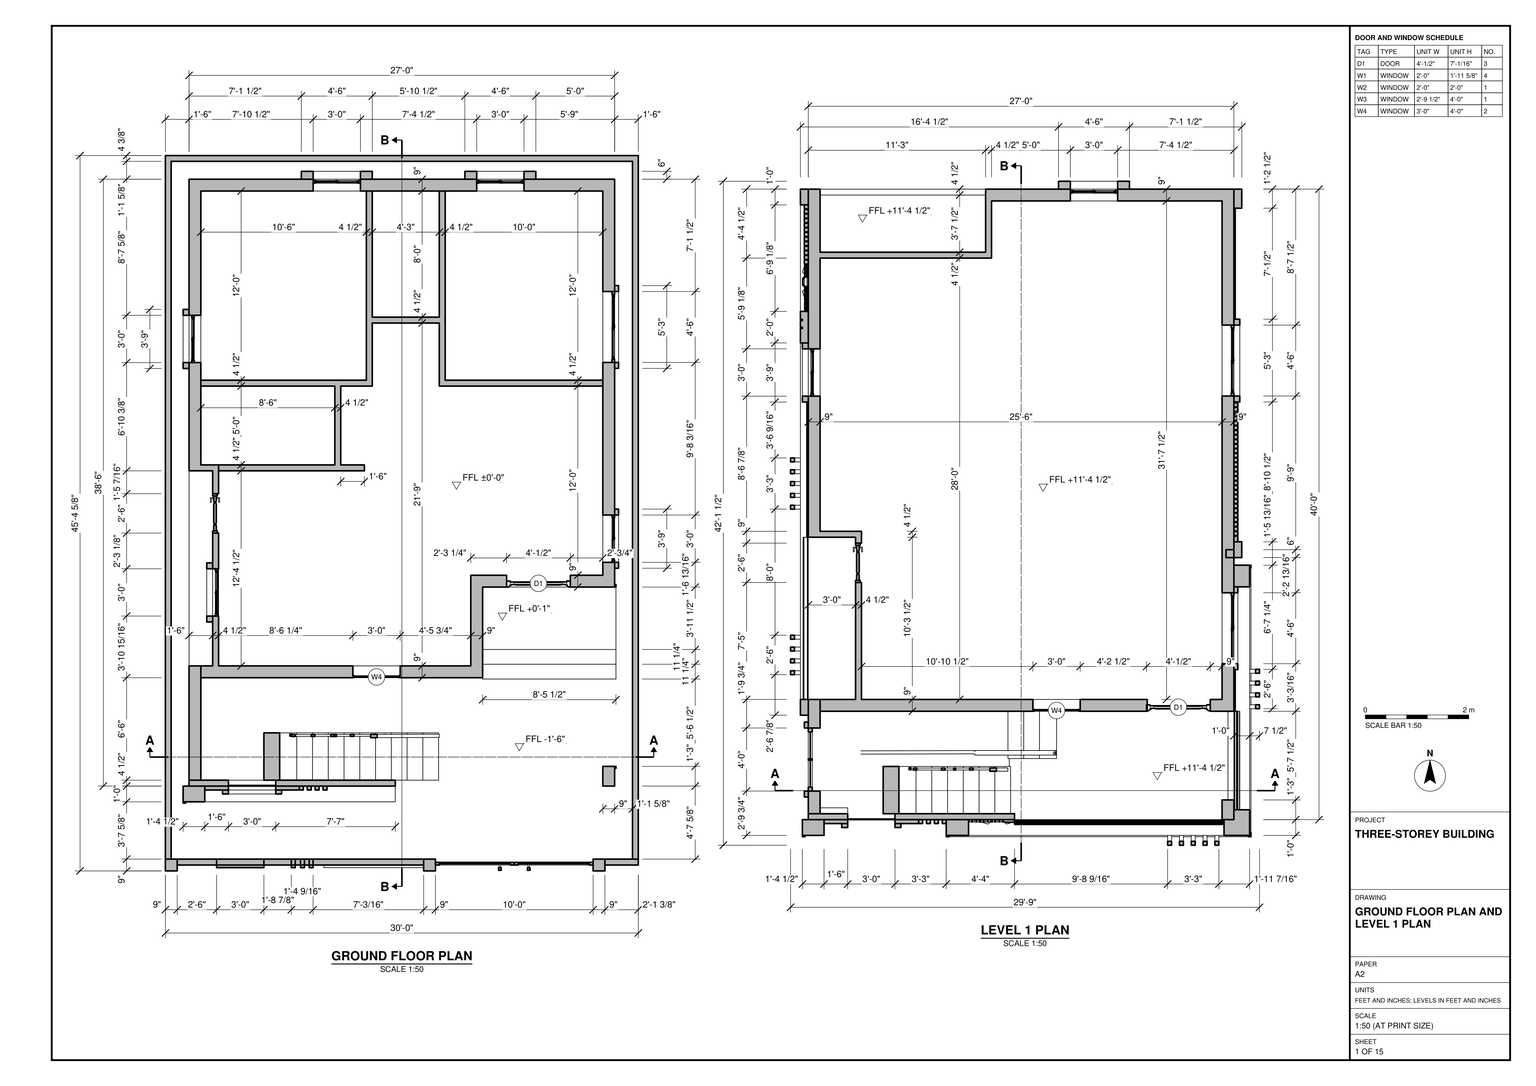
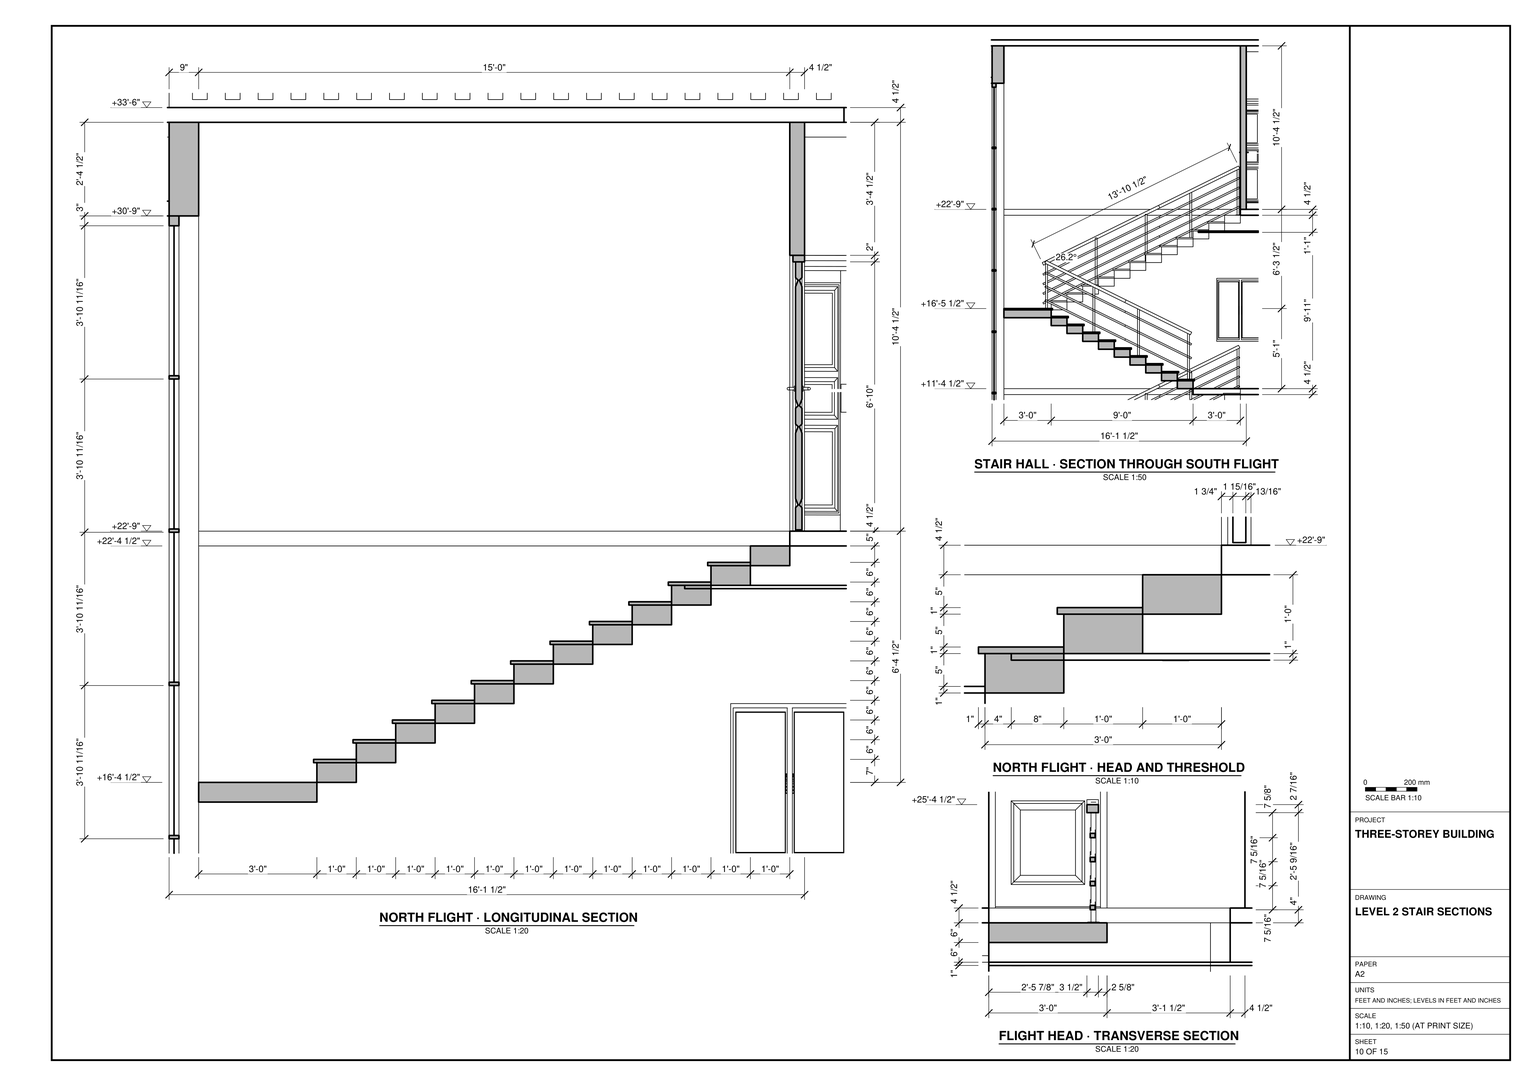
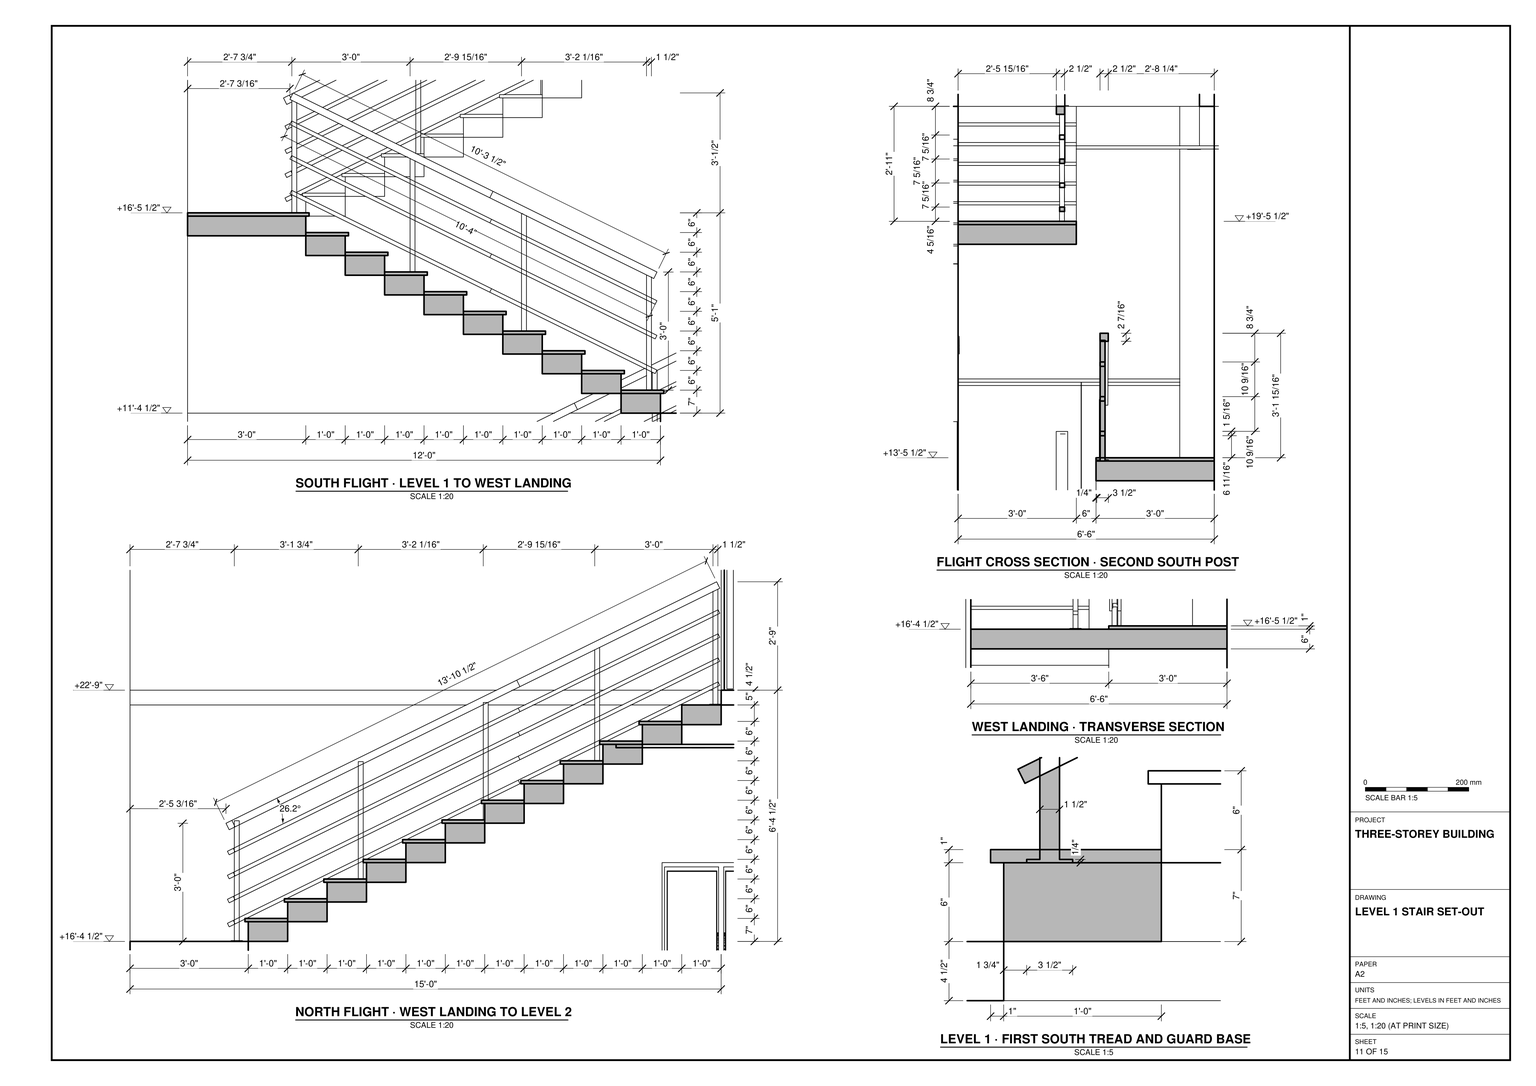
Build the three-storey building in SketchUp from task_files/diagram_01.pdf. Work in feet and inches. The complete model, including projections, must measure 30'-2 7/8" along X, 46'-9 1/8" along Y and 37'-11 1/16" along Z. Set the finished floor levels to ±0'-0" at ground level, +11'-4 1/2" at Level 1 and +22'-9" at Level 2.

Follow each floor plan separately. On the ground floor, form the larger rooms on either side of the narrow rear space, the smaller enclosure on the left and the stepped entrance on the right. On Level 1, retain the broad open floor area and the offsets in its enclosing walls. Model the walls at their drawn thicknesses, the floor slabs and their projecting edges, the supports, the roof and the framed door and window openings. Use the stair plans and sections together: connect the flights through their landings, form the individual treads and carry the guards up the slopes to the flight heads. Include built-in joinery and main furniture where shown. Any decor or loose items shown may use suitable library components.

Keep walls, slabs, roof elements and individual furniture or joinery pieces in separate groups or components, and use components for repeated parts. Save one SketchUp model as output_files/three_storey_building_with_its_return_stair.skp.

# SketchUp Ruby script. Lengths in inches.
U = 1.inch
M = Sketchup.active_model
def pt(a) = Geom::Point3d.new(a.map { |v| v * U })
def face(e, loops, mat)
  f = e.add_face(loops[0].map { |a| pt(a) })
  loops[1..].each { |l| e.add_face(l.map { |a| pt(a) }).erase! }
  f.material = f.back_material = mat if mat
  f
end
# faces: each face lists its corners as indices into pts; further lists are holes
def faces(e, pts, list, mat = nil) = list.each { |f| face(e, (f[0].is_a?(Array) ? f : [f]).map { |l| l.map { |i| pts[i] } }, mat) }
# xy, xz, yz: faces in a plane at the given z, y or x. An outline is a flat list of corners, or four numbers for a rectangle; further outlines are holes
def ring(l) = l.size == 4 ? [[l[0], l[1]], [l[2], l[1]], [l[2], l[3]], [l[0], l[3]]] : l.each_slice(2).to_a
def flat(e, list, mat, &to3) = list.each { |f| face(e, (f[0].is_a?(Array) ? f : [f]).map { |l| ring(l).map { |u, v| to3.(u, v) } }, mat) }
def xy(e, z, list, mat = nil) = flat(e, list, mat) { |x, y| [x, y, z] }
def xz(e, y, list, mat = nil) = flat(e, list, mat) { |x, z| [x, y, z] }
def yz(e, x, list, mat = nil) = flat(e, list, mat) { |y, z| [x, y, z] }
def lines(e, pts, list) = list.each { |a, b| e.add_line(pt(pts[a]), pt(pts[b])) }
# prism: a flat outline (further loops are holes) pulled along v
def prism(e, loops, v, mat = nil)
  f = face(e, loops, mat); d = Geom::Vector3d.new(v.map { |x| x * U })
  f.pushpull(f.normal.samedirection?(d) ? d.length : -d.length)
end
def box(e, o, s, mat = nil) = prism(e, [[o, [o[0] + s[0], o[1], o[2]], [o[0] + s[0], o[1] + s[1], o[2]], [o[0], o[1] + s[1], o[2]]]], [0, 0, s[2]], mat)
def at(x, y, z, deg = 0) = Geom::Transformation.translation(pt([x, y, z])) * Geom::Transformation.rotation(ORIGIN, Z_AXIS, deg.degrees)
def axes(o, x, y, z) = Geom::Transformation.new([*x, 0, *y, 0, *z, 0, *pt(o).to_a, 1])
def part(name) = M.definitions.add(name)
# library, detail: a bought-in or finely detailed component or shape, given as its bounding box
def library(name, o, s) = part(name).tap { |d| box(d.entities, o, s) }
def detail(e, o, s) = box(e.add_group.entities, o, s)
def put(e, d, t, mat = nil) = e.add_instance(d, t).tap { |i| i.material = mat if mat }
def group(e, t, mat = nil) = e.add_group.tap { |g| g.transformation = t; g.material = mat if mat }.entities
root = M.entities
M.materials.add("[0042_Sienna]").color = [131, 75, 41]
M.materials.add("[0043_SaddleBrown]").color = [139, 69, 19]
M.materials.add("[Carrera Marble]").color = [207, 207, 207]
M.materials.add("[Color A01]").color = [116, 113, 107]
M.materials.add("[Color A01]1").color = [209, 202, 182]
M.materials.add("[Color A02]").color = [191, 184, 171]
M.materials.add("[Color A02]3").color = [191, 184, 171]
M.materials.add("[Color A07]").color = [198, 120, 50]
M.materials.add("[Color L05]").color = [255, 255, 255]
M.materials.add("[Color M00]").color = [255, 255, 255]
M.materials.add("[Color M05]").color = [114, 114, 114]
M.materials.add("[Color M08]").color = [30, 30, 30]
M.materials.add("[Concrete Aggregate Smoke]").color = [154, 150, 148]
M.materials.add("[Translucent Glass Gray]").color = [128, 128, 128]
M.materials["[Translucent Glass Gray]"].alpha = 0.5
c1 = library("Porta_Principal_Aluminio_1,7_double door",[0,-2.5625,-0.08],[70.55,6.25,84.08])
c2 = library("Window",[76.48,18.9,0],[35.3,2.01,48])
c3 = library("ventilator\#1",[0,0,0],[24,6.83,23.62])
c4 = library("Group\#54",[0,0,-18],[181,78,151])
c5 = library("Group\#233",[0,0,0],[2,48,48])
c6 = part("Group\#64")
prism(c6.entities,[[[0,54,66],[0,54,0],[0,0,0],[0,0,66]],[[0,45,9],[0,45,57],[0,9,57],[0,9,9]]],[6,0,0])
c7 = part("Group\#52")
box(c7.entities,[0,0,0],[324,4.5,36])
c8 = part("Group\#55")
box(c8.entities,[0,0,0],[4.5,265.5,36])
c9 = part("Group\#254")
box(c9.entities,[0,0,1.0625],[10,4.5,10])
c10 = library("Group\#186",[0,0,0],[11.5625,11.5625,14.875])
c11 = library("Group\#185",[0,0,0],[11.5625,11.5625,14.875])
c12 = library("Group\#354",[74.9375,-1,-1],[75,4,37])
c13 = part("Group155\#2")
xy(c13.entities,0,[[-21,-139.5,-0.5,-93.83],[0.5,-139.5,21,-93.83],[-21,-92.83,-0.5,-47.17],[0.5,-92.83,21,-47.17],[-21,-46.17,-0.5,-0.5],
  [0.5,-46.17,21,-0.5],[-21,0.5,-0.5,46.17],[0.5,0.5,21,46.17],[-21,47.17,-0.5,92.83],[0.5,47.17,21,92.83],
  [-21,93.83,-0.5,139.5],[0.5,93.83,21,139.5]])
c14 = part("Group154\#1")
prism(c14.entities,[[[24,142.5,0],[24,-142.5,0],[-24,-142.5,0],[-24,142.5,0]],[[-0.5,46.17,0],[-21,46.17,0],[-21,0.5,0],[-0.5,0.5,0]],[[-0.5,47.17,0],[-0.5,92.83,0],[-21,92.83,0],[-21,47.17,0]],[[-21,-92.83,0],[-0.5,-92.83,0],[-0.5,-47.17,0],[-21,-47.17,0]],[[-0.5,-93.83,0],[-21,-93.83,0],[-21,-139.5,0],[-0.5,-139.5,0]],[[-21,-0.5,0],[-21,-46.17,0],[-0.5,-46.17,0],[-0.5,-0.5,0]],[[-0.5,93.83,0],[-0.5,139.5,0],[-21,139.5,0],[-21,93.83,0]],[[0.5,92.83,0],[0.5,47.17,0],[21,47.17,0],[21,92.83,0]],[[21,46.17,0],[0.5,46.17,0],[0.5,0.5,0],[21,0.5,0]],[[21,93.83,0],[21,139.5,0],[0.5,139.5,0],[0.5,93.83,0]],[[21,-0.5,0],[0.5,-0.5,0],[0.5,-46.17,0],[21,-46.17,0]],[[21,-92.83,0],[21,-47.17,0],[0.5,-47.17,0],[0.5,-92.83,0]],[[0.5,-93.83,0],[0.5,-139.5,0],[21,-139.5,0],[21,-93.83,0]]],[0,0,3])
put(c14.entities,c13,at(0,0,1.5),"[Translucent Glass Gray]")
c15 = library("Group\#197",[0,0,0],[127.37,119.9375,0.1])
c16 = library("Group\#81",[-65.34,0,-23.05],[151.15,3.75,160.05])
c17 = library("Group\#46",[0,0,0],[180,78,132])
c18 = library("Group\#61",[0,0,0],[193.5,4.5,415.5])
c19 = library("Group\#123",[0,0,0],[101.5,70,19])
c20 = part("Group\#97")
box(c20.entities,[0,0,0],[9,8.92,124.5])
c21 = part("Group\#31")
box(c21.entities,[0,0,0],[3,3,330])
c22 = library("Group\#284",[23.9375,-1,-1],[126,4,37])
c23 = part("Group\#69")
xy(c23.entities,0,[[0,0,3,7.5]])
xy(c23.entities,3,[[0,3,3,7.5]])
xy(c23.entities,124.5,[[0,3,3,7.5]])
xy(c23.entities,127.5,[[0,0,3,3],[0,3,3,7.5]])
xz(c23.entities,0,[[0,0,3,127.5]])
xz(c23.entities,3,[[0,3,3,124.5],[0,124.5,3,127.5]])
xz(c23.entities,7.5,[[0,0,3,3],[0,124.5,3,127.5]])
yz(c23.entities,0,[[0,0,0,127.5,3,127.5,3,3,7.5,3,7.5,0],[3,124.5,7.5,127.5]])
yz(c23.entities,3,[[0,0,7.5,0,7.5,3,3,3,3,127.5,0,127.5],[3,124.5,7.5,127.5]])
c24 = part("Group\#152")
xy(c24.entities,-113.04,[[0,0,3,7.5]])
xy(c24.entities,-110.04,[[0,3,3,7.5]])
xy(c24.entities,124.5,[[0,3,3,7.5]])
xy(c24.entities,127.5,[[0,0,3,3],[0,3,3,7.5]])
xz(c24.entities,0,[[0,-113.04,3,127.5]])
xz(c24.entities,3,[[0,-110.04,3,124.5],[0,124.5,3,127.5]])
xz(c24.entities,7.5,[[0,-113.04,3,-110.04],[0,124.5,3,127.5]])
yz(c24.entities,0,[[0,-113.04,0,127.5,3,127.5,3,-110.04,7.5,-110.04,7.5,-113.04],[3,124.5,7.5,127.5]])
yz(c24.entities,3,[[0,-113.04,7.5,-113.04,7.5,-110.04,3,-110.04,3,127.5,0,127.5],[3,124.5,7.5,127.5]])
c25 = part("Group\#113")
box(c25.entities,[0,-1,0],[2,3,9])
c26 = library("Group\#242",[0,0,0],[7.09,35.43,83.07])
c27 = part("Group\#245")
prism(c27.entities,[[[4.5,33,33],[4.5,0,33],[4.5,0,0],[4.5,33,0]],[[4.5,28.5,28.5],[4.5,28.5,4.5],[4.5,4.5,4.5],[4.5,4.5,28.5]]],[-4.5,0,0])
c28 = part("Group\#232")
box(c28.entities,[0,0,0],[1,31.72,6])
c29 = part("Group\#230")
box(c29.entities,[0,0,0],[1,94.72,6])
c30 = library("Group\#248",[0,0,12],[3,45,277.5])
c31 = part("Group\#256")
put(c31.entities,c23,at(36,0,0),"[Color M08]")
put(c31.entities,c23,at(18,0,0),"[Color M08]")
put(c31.entities,c23,at(27,0,0),"[Color M08]")
put(c31.entities,c23,at(9,0,0),"[Color M08]")
c32 = library("Group\#94",[0,0,0],[128.5,100.5,4.5])
c33 = library("Group\#59",[38.9375,-1,-1],[111,4,37])
c34 = library("Group\#264",[0,0,0],[35,3.375,108])
c35 = library("Group\#323",[0,35,0],[3.375,35,135])
c36 = library("Group\#198",[0,0,0],[127.37,66.875,0.1])
c37 = library("Group\#372",[0,0,0],[1,147.9,130])
c38 = library("VASANTHA HOUSE",[0.32,0,0],[80.88,5.5,1])
c39 = part("Group\#155")
box(c39.entities,[0,0,0],[9,9,90])
c40 = part("Group\#156")
box(c40.entities,[33,0,0],[3,6.5,90])
c41 = library("Group\#208",[0,0,0],[59.75,6,78])
c42 = library("Group\#175",[0,0,0],[59.75,6,78])
c43 = library("Group\#252",[-9.5625,-1,-1],[159.5,4,37])
c44 = library("Group\#82",[-65.34,0,-23.05],[151.15,3.75,160.05])
c45 = library("Group\#216",[0,0,0],[36,0.5,327])
c46 = library("Group\#253",[-0.67,-1.3,-4.8125],[36.06,79.87,6.15])
c47 = library("Group\#80",[-65.34,0,3.58],[112.56,3.75,126.32])
c48 = library("Group\#334",[0,6,0],[3,169.5,289.5])
put(root,c1,axes([201,284.88,291],[0.68725,0,0],[0,1,0],[0,0,1]))
put(root,c1,axes([259.76,228.88,18],[0.68725,0,0],[0,1,0],[0,0,1]))
put(root,c2,axes([49.71,264.7,327],[0.94892,0,0],[0,1,0],[0,0,1]))
put(root,c3,axes([18,349.6,238.5],[0,-1,0],[1,0,0],[0,0,1.016]),"[Color A02]")
put(root,c2,axes([64.75,138.22,54],[1.01974,0,0],[0,1,0],[0,0,1]))
put(root,c1,axes([275.51,160.16,154.58],[0.68725,0,0],[0,1,0],[0,0,1]))
put(root,c3,at(18,349.6,102,-90))
put(root,c2,axes([111.01,138.22,190.5],[1.01974,0,0],[0,1,0],[0,0,1]))
g1 = group(root,at(342,268.82,150),"[Color A02]3")
xy(g1,0,[[0,187.28,1,245.76]],"[Color A02]3")
xy(g1,289.5,[[0,187.28,1,245.76]],"[Color A02]3")
xz(g1,187.28,[[0,0,1,36],[0,36,1,172.5],[0,172.5,1,229.5],[0,229.5,1,289.5]],"[Color A02]3")
xz(g1,245.76,[[0,0,1,172.5],[0,172.5,1,229.5],[0,229.5,1,289.5]],"[Color A02]3")
yz(g1,0,[[187.28,229.5,245.76,289.5]],"[Color A02]3")
yz(g1,1,[[187.28,0,245.76,289.5]],"[Color A02]3")
put(root,c4,at(27,79.6,18))
g2 = group(root,at(241.5,84.1,137),"[Color A07]")
prism(g2,[[[0,142.5,0],[91.5,142.5,0],[91.5,0,0],[-46.5,0,0],[-46.5,73.5,0],[0,73.5,0]]],[0,0,1])
g3 = group(root,at(18,79.6,18),"[Color A02]")
prism(g3,[[[0,87,0],[0,0,0],[0,0,397.5],[0,87,397.5]],[[0,17.25,369],[0,17.25,84],[0,65.25,84],[0,65.25,369]]],[9,0,0])
g4 = group(root,at(342,514.57,150))
box(g4,[0,0,0],[1,26.03,289.5])
g5 = group(root,at(12,75.1,18))
put(g5,c3,at(159.85,473.17,357))
put(g5,c3,at(157.5,455.17,84))
put(g5,c3,at(156.85,473.17,220.5))
g6 = group(g5,at(6,82.5,0))
xy(g6,0,[[9,0,9,9,18,9,18,110.09,22.5,110.09,22.5,9,214.5,9,214.5,78,241.77,78,241.77,69,223.5,69,223.5,0],[290.25,69,290.25,78,315,78,315,370.5,9,370.5,9,162,22.5,162,22.5,140.09,18,140.09,18,157.5,0,157.5,0,379.5,324,379.5,324,69]])
xy(g6,36,[[124.73,0,160.73,9],[18,46.93,22.5,82.93],[315,87.84,324,123.84],[0,239.9,9,275.9],[315,240,324,294],
  [94.5,370.5,130.5,379.5],[219,370.5,255,379.5]])
xy(g6,84,[[124.73,0,160.73,9],[18,46.93,22.5,82.93],[241.77,69,290.25,78],[315,87.84,324,123.84],[18,110.09,22.5,140.09],
  [0,168,9,192],[0,239.9,9,275.9],[315,240,324,294],[94.5,370.5,130.5,379.5],[150.85,370.5,175.5,379.5],
  [219,370.5,255,379.5]])
xy(g6,108,[[0,168,9,192],[150.85,370.5,175.5,379.5]])
xy(g6,132,[[[9,0,223.5,0,223.5,69,324,69,324,379.5,0,379.5,0,157.5,18,157.5,18,9,9,9],[22.5,9,22.5,162,9,162,9,370.5,315,370.5,315,78,214.5,78,214.5,9]]])
xz(g6,0,[[[9,0,223.5,132],[124.73,36,160.73,84]]],"[Carrera Marble]")
xz(g6,9,[[9,0,18,132],[[22.5,0,214.5,132],[124.73,36,160.73,84]]])
xz(g6,46.93,[[18,36,22.5,84]])
xz(g6,69,[[223.5,0,241.77,0,241.77,84,290.25,84,290.25,0,324,0,324,132,223.5,132]],"[Carrera Marble]")
xz(g6,78,[[214.5,0,214.5,132,315,132,315,0,290.25,0,290.25,84,241.77,84,241.77,0]])
xz(g6,82.93,[[18,36,22.5,84]])
xz(g6,87.84,[[315,36,324,84]])
xz(g6,110.09,[[18,0,22.5,84]])
xz(g6,123.84,[[315,36,324,84]])
xz(g6,140.09,[[18,0,22.5,84]])
xz(g6,157.5,[[0,0,18,132]])
xz(g6,162,[[9,0,22.5,132]])
xz(g6,168,[[0,84,9,108]])
xz(g6,192,[[0,84,9,108]])
xz(g6,239.9,[[0,36,9,84]])
xz(g6,240,[[315,36,324,84]])
xz(g6,275.9,[[0,36,9,84]])
xz(g6,294,[[315,36,324,84]])
xz(g6,370.5,[[[9,0,315,132],[94.5,36,130.5,84],[219,36,255,84],[150.85,84,175.5,108]]])
xz(g6,379.5,[[[0,0,324,132],[219,36,255,84],[94.5,36,130.5,84],[150.85,84,175.5,108]]])
yz(g6,0,[[[157.5,0,379.5,132],[239.9,36,275.9,84],[168,84,192,108]]])
yz(g6,9,[[0,0,9,132],[[162,0,370.5,132],[239.9,36,275.9,84],[168,84,192,108]]])
yz(g6,18,[[[9,0,9,132,157.5,132,157.5,0,140.09,0,140.09,84,110.09,84,110.09,0],[46.93,36,82.93,84]]])
yz(g6,22.5,[[[9,0,110.09,0,110.09,84,140.09,84,140.09,0,162,0,162,132,9,132],[46.93,36,82.93,84]]])
yz(g6,94.5,[[370.5,36,379.5,84]])
yz(g6,124.73,[[0,36,9,84]])
yz(g6,130.5,[[370.5,36,379.5,84]])
yz(g6,150.85,[[370.5,84,379.5,108]])
yz(g6,160.73,[[0,36,9,84]])
yz(g6,175.5,[[370.5,84,379.5,108]])
yz(g6,214.5,[[9,0,78,132]])
yz(g6,219,[[370.5,36,379.5,84]])
yz(g6,223.5,[[0,0,69,132]],"[Carrera Marble]")
yz(g6,241.77,[[69,0,78,84]])
yz(g6,255,[[370.5,36,379.5,84]])
yz(g6,290.25,[[69,0,78,84]])
yz(g6,315,[[[78,0,370.5,132],[240,36,294,84],[87.84,36,123.84,84]]])
yz(g6,324,[[[69,0,379.5,132],[240,36,294,84],[87.84,36,123.84,84]]])
put(g5,c5,axes([136.5,459,36],[0,1,0],[-0.75,0,0],[0,0,1]))
g7 = group(g5,at(153.78,199.5,300,90))
prism(g7,[[[1.5,49.5,61.5],[1.5,49.5,4.5],[1.5,4.5,4.5],[1.5,4.5,61.5]],[[1.5,45,9],[1.5,45,57],[1.5,9,57],[1.5,9,9]]],[4.5,0,0])
g8 = group(g5,at(18,120.43,27))
prism(g8,[[[1.5,49.5,61.5],[1.5,49.5,4.5],[1.5,4.5,4.5],[1.5,4.5,61.5]],[[1.5,45,9],[1.5,45,57],[1.5,9,57],[1.5,9,9]]],[4.5,0,0])
put(g5,c6,at(270,462,27.14,90))
put(g5,c7,at(6,205.5,397.5))
put(g5,c7,at(6,475.5,397.5))
put(g5,c8,at(325.5,210,397.5))
put(g5,c8,at(6,210,397.5))
put(g5,c5,axes([136.5,477,309],[0,1,0],[-0.75,0,0],[0,0,1]))
put(g5,c5,axes([241.5,477,172.5],[0,1,0],[-0.75,0,0],[0,0,1]))
g9 = group(g5,at(6,205.5,273))
xy(g9,0,[[231.49,0,231.49,9,315,9,315,265.5,9,265.5,9,121.5,37.5,121.5,37.5,112.42,33,112.42,33,117,0,117,0,274.5,324,274.5,324,0],[33,0,33,82.42,37.5,82.42,37.5,9,183.49,9,183.49,0]])
xy(g9,36,[[104.28,0,137.78,9],[33,58.79,37.5,76.79],[315,117,324,171],[0,125.25,9,161.25],[94.5,265.5,130.5,274.5]])
xy(g9,84,[[104.28,0,137.78,9],[183.49,0,231.49,9],[33,58.79,37.5,76.79],[33,82.42,37.5,112.42],[315,117,324,171],
  [0,125.25,9,161.25],[94.5,265.5,130.5,274.5],[153.85,265.5,177.85,274.5]])
xy(g9,108,[[153.85,265.5,177.85,274.5]])
xy(g9,120,[[[33,0,324,0,324,274.5,0,274.5,0,117,33,117],[37.5,9,37.5,121.5,9,121.5,9,265.5,315,265.5,315,9]]])
xz(g9,0,[[[33,0,183.49,0,183.49,84,231.49,84,231.49,0,324,0,324,120,33,120],[104.28,36,137.78,84]]])
xz(g9,9,[[[37.5,0,37.5,120,315,120,315,0,231.49,0,231.49,84,183.49,84,183.49,0],[104.28,36,137.78,84]]])
xz(g9,58.79,[[33,36,37.5,84]])
xz(g9,76.79,[[33,36,37.5,84]])
xz(g9,82.42,[[33,0,37.5,84]])
xz(g9,112.42,[[33,0,37.5,84]])
xz(g9,117,[[315,36,324,84]])
xz(g9,117,[[0,0,33,120]],"[Carrera Marble]")
xz(g9,121.5,[[9,0,37.5,120]])
xz(g9,125.25,[[0,36,9,84]])
xz(g9,161.25,[[0,36,9,84]])
xz(g9,171,[[315,36,324,84]])
xz(g9,229.47,[[315,36,324,84],[315,36,324,84]])
xz(g9,265.5,[[[9,0,315,120],[94.5,36,130.5,84],[153.85,84,177.85,108]]])
xz(g9,274.5,[[[0,0,324,120],[94.5,36,130.5,84],[153.85,84,177.85,108]]])
yz(g9,0,[[[117,0,274.5,120],[125.25,36,161.25,84]]])
yz(g9,9,[[[121.5,0,265.5,120],[125.25,36,161.25,84]]])
yz(g9,33,[[[0,0,0,120,117,120,117,0,112.42,0,112.42,84,82.42,84,82.42,0],[58.79,36,76.79,84]]],"[Carrera Marble]")
yz(g9,37.5,[[[9,0,82.42,0,82.42,84,112.42,84,112.42,0,121.5,0,121.5,120,9,120],[58.79,36,76.79,84]]])
yz(g9,94.5,[[265.5,36,274.5,84]])
yz(g9,104.28,[[0,36,9,84]])
yz(g9,130.5,[[265.5,36,274.5,84]])
yz(g9,137.78,[[0,36,9,84]])
yz(g9,153.85,[[265.5,84,274.5,108]])
yz(g9,177.85,[[265.5,84,274.5,108]])
yz(g9,183.49,[[0,0,9,84]])
yz(g9,231.49,[[0,0,9,84]])
yz(g9,315,[[[9,0,265.5,120],[117,36,171,84]]])
yz(g9,324,[[[0,0,274.5,120],[117,36,171,84]]])
g10 = group(g5,at(6,0,136.5))
xy(g10,0,[[306,82.5,306,91.5,315,91.5,315,471,139.5,471,139.5,427.5,9,427.5,9,219.5,40.5,219.5,40.5,210.5,36,210.5,36,215,0,215,0,480,9,480,9,432,135,432,135,480,324,480,324,82.5],[9,82.5,9,91.5,36,91.5,36,180.5,40.5,180.5,40.5,91.5,258,91.5,258,82.5]])
xy(g10,36,[[171,82.5,207,91.5],[315,118.72,324,172.72],[0,322.4,9,358.4],[315,322.5,324,376.5],[199.5,471,235.5,480]])
xy(g10,84,[[171,82.5,207,91.5],[258,82.5,306,91.5],[315,118.72,324,172.72],[36,180.5,40.5,210.5],[0,250.5,9,274.5],
  [0,322.4,9,358.4],[315,322.5,324,376.5],[150.85,471,174.85,480],[199.5,471,235.5,480]])
xy(g10,108,[[0,250.5,9,274.5],[150.85,471,174.85,480]])
xy(g10,132,[[[9,82.5,324,82.5,324,480,135,480,135,432,9,432,9,480,0,480,0,215,36,215,36,91.5,9,91.5],[40.5,91.5,40.5,219.5,9,219.5,9,427.5,139.5,427.5,139.5,471,315,471,315,91.5]]])
xz(g10,82.5,[[[9,0,258,0,258,84,306,84,306,0,324,0,324,132,9,132],[171,36,207,84]]],"[Carrera Marble]")
xz(g10,91.5,[[9,0,36,132],[[40.5,0,40.5,132,315,132,315,0,306,0,306,84,258,84,258,0],[171,36,207,84]]])
xz(g10,118.72,[[315,36,324,84]])
xz(g10,172.72,[[315,36,324,84]])
xz(g10,180.5,[[36,0,40.5,84]])
xz(g10,210.5,[[36,0,40.5,84]])
xz(g10,215,[[0,0,36,132]],"[Carrera Marble]")
xz(g10,219.5,[[9,0,40.5,132]])
xz(g10,250.5,[[0,84,9,108]])
xz(g10,274.5,[[0,84,9,108]])
xz(g10,322.4,[[0,36,9,84]])
xz(g10,322.5,[[315,36,324,84]])
xz(g10,358.4,[[0,36,9,84]])
xz(g10,376.5,[[315,36,324,84]])
xz(g10,427.5,[[9,0,139.5,132]])
xz(g10,432,[[9,0,135,132]])
xz(g10,471,[[[139.5,0,315,132],[199.5,36,235.5,84],[150.85,84,174.85,108]]])
xz(g10,480,[[0,0,9,132],[[135,0,324,132],[199.5,36,235.5,84],[150.85,84,174.85,108]]])
yz(g10,0,[[[215,0,480,132],[322.4,36,358.4,84],[250.5,84,274.5,108]]])
yz(g10,9,[[82.5,0,91.5,132],[[219.5,0,427.5,132],[322.4,36,358.4,84],[250.5,84,274.5,108]],[432,0,480,132]])
yz(g10,36,[[91.5,0,91.5,132,215,132,215,0,210.5,0,210.5,84,180.5,84,180.5,0]],"[Carrera Marble]")
yz(g10,40.5,[[91.5,0,180.5,0,180.5,84,210.5,84,210.5,0,219.5,0,219.5,132,91.5,132]])
yz(g10,135,[[432,0,480,132]])
yz(g10,139.5,[[427.5,0,471,132]])
yz(g10,150.85,[[471,84,480,108]])
yz(g10,171,[[82.5,36,91.5,84]])
yz(g10,174.85,[[471,84,480,108]])
yz(g10,199.5,[[471,36,480,84]])
yz(g10,207,[[82.5,36,91.5,84]])
yz(g10,235.5,[[471,36,480,84]])
yz(g10,258,[[82.5,0,91.5,84]])
yz(g10,306,[[82.5,0,91.5,84]])
yz(g10,315,[[[91.5,0,471,132],[118.72,36,172.72,84],[322.5,36,376.5,84]]])
yz(g10,324,[[[82.5,0,480,132],[118.72,36,172.72,84],[322.5,36,376.5,84]]])
p = [[324,0,0],[324,4.5,0],[319.5,82.5,0],[319.5,4.5,0]]
lines(g10,p,[[0,1],[2,3]])
put(g5,c5,axes([28,165.43,36],[-1,0,0],[0,-0.75,0],[0,0,1]))
put(g5,c5,axes([10,366.75,309],[-1,0,0],[0,-0.75,0],[0,0,1]))
put(g5,c5,axes([328,322.5,36],[1,0,0],[0,1.125,0],[0,0,1]))
put(g5,c5,axes([328,170.34,36],[1,0,0],[0,0.75,0],[0,0,1]))
put(g5,c5,axes([261,459,36],[0,1,0],[-0.75,0,0],[0,0,1]))
put(g5,c6,at(145.5,479,300,90))
put(g5,c6,at(145.5,462,27.14,90))
put(g5,c6,at(250.5,480,163.5,90))
put(g5,c5,axes([328,118.72,172.5],[1,0,0],[0,1.125,0],[0,0,1]))
g11 = group(root,at(41.62,269.6,422.43,90))
put(g11,c9,at(0,2,-1.0625))
put(g11,c9,at(0,12,-1.0625))
put(g11,c9,at(0,-8,-1.0625))
put(g11,c9,at(0,-18,-1.0625))
put(g11,c9,at(0,-28,-1.0625))
put(g11,c9,at(0,-38,-1.0625))
put(g11,c9,at(0,-48,-1.0625))
put(g11,c9,at(0,-58,-1.0625))
put(g11,c9,at(0,-68,-1.0625))
put(g11,c9,at(0,-78,-1.0625))
put(g11,c9,at(0,-88,-1.0625))
put(g11,c9,at(0,-98,-1.0625))
put(g11,c9,at(0,-108,-1.0625))
put(g11,c9,at(0,-118,-1.0625))
put(g11,c9,at(0,-128,-1.0625))
put(g11,c9,at(0,-138,-1.0625))
put(g11,c9,at(0,-148,-1.0625))
put(g11,c9,at(0,-158,-1.0625))
put(g11,c9,at(0,-168,-1.0625))
put(g11,c9,at(0,-178,-1.0625))
g12 = group(root,at(211.5,75.1,154.5))
box(g12,[-184.5,475.5,0],[126,4.5,42])
g13 = group(root,at(12,388.5,45))
prism(g13,[[[1.5,49.5,61.5],[1.5,49.5,4.5],[1.5,4.5,4.5],[1.5,4.5,61.5]],[[1.5,45,9],[1.5,45,57],[1.5,9,57],[1.5,9,9]]],[4.5,0,0])
g14 = group(root,at(-1.375,9,90))
put(g14,c10,at(196.6,0,0))
put(g14,c11,at(325.6,0,0))
put(g14,c10,at(0,0,0))
g15 = group(root,at(196.6,0,-1),"[Concrete Aggregate Smoke]")
box(g15,[0,0,0],[138,19.5,1])
g16 = group(root,at(223.5,62.1,417))
xy(g16,1,[[0,0,0,1,133,1,133,107.5,134,107.5,134,0]])
xy(g16,3,[[0,0,133,1],[133,0,134,107.5]])
xz(g16,0,[[0,1,134,3]])
xz(g16,1,[[0,1,133,3]])
xz(g16,107.5,[[133,1,134,3]])
yz(g16,0,[[0,1,1,3]])
yz(g16,133,[[1,1,107.5,3]])
yz(g16,134,[[0,1,107.5,3]])
g17 = group(root,at(241.5,84.1,268.5),"[Color A07]")
prism(g17,[[[0,73.5,5],[100.5,73.5,5],[100.5,-9,5],[-66.5,-9,5],[-66.5,73.5,5]]],[0,0,1])
put(root,c12,at(343.5,232.54,167.5,-90))
g18 = group(root,at(18,280.6,291))
xy(g18,0,[[189,-201.08,193.5,-159],[9,-123,193.5,-114]])
xy(g18,84,[[189,-159,193.5,-123]])
xy(g18,124.5,[[189,-201.08,193.5,-201.08,193.5,-114,9,-114,9,-123,189,-123]])
xz(g18,-201.08,[[189,0,193.5,124.5]])
xz(g18,-159,[[189,0,193.5,84]])
xz(g18,-123,[[9,0,189,124.5],[189,0,193.5,84]])
xz(g18,-114,[[9,0,193.5,124.5]])
yz(g18,9,[[-123,0,-114,124.5]])
yz(g18,189,[[-201.08,0,-201.08,124.5,-123,124.5,-123,84,-159,84,-159,0]])
yz(g18,193.5,[[-201.08,0,-159,0,-159,84,-123,84,-123,0,-114,0,-114,124.5,-201.08,124.5]])
g19 = group(g18,at(37.5,117,0))
prism(g19,[[[102,48,0],[102,0,0],[0,0,0],[0,4.5,0],[97.5,4.5,0],[97.5,148.5,0],[102,148.5,0],[102,52.5,0],[156,52.5,0],[156,148.5,0],[160.5,148.5,0],[160.5,48,0]]],[0,0,120])
g20 = group(root,at(18,280.6,411))
box(g20,[0,0,0],[324,274.5,4.5])
g21 = group(root,at(333,90.1,274.5))
box(g21,[0,0,0],[9,67.5,12])
put(root,c14,axes([21,120.85,244.5],[0,-1,0],[0,0,1],[-1,0,0]),"[Color M08]")
put(root,c15,at(198.04,95.75,136.9))
put(root,c16,at(141.66,127.72,78,180))
g22 = group(root,at(342,240.9375,49.5))
prism(g22,[[[3,0,57],[3,0,0],[3,45,0],[3,45,57]],[[3,40.5,4.5],[3,4.5,4.5],[3,4.5,52.5],[3,40.5,52.5]]],[-3,0,0])
g23 = group(root,at(18,75.1,150))
prism(g23,[[[157,4.5,0],[66,4.5,0],[66,9,0],[153,9,0],[153,46.5,0],[189,46.5,0],[189,82.5,0],[9,82.5,0],[9,91.5,0],[0,91.5,0],[0,480,0],[324,480,0],[324,0,0],[157,0,0]]],[0,0,4.5])
box(g23,[9,4.5,0],[21,4.5,4.5])
put(root,c17,at(27,79.6,154.5))
g24 = group(root,at(37.5,69.1,304.5))
xy(g24,-249,[[6,0,51,3]])
xy(g24,-244.5,[[10.5,0,46.5,3]])
xy(g24,82.5,[[10.5,0,46.5,3]])
xy(g24,87,[[6,0,51,3]])
xz(g24,0,[[[6,-249,51,87],[10.5,-244.5,46.5,82.5]]])
xz(g24,3,[[6,-249,6,87,51,87,51,-244.5,46.5,-244.5,46.5,82.5,10.5,82.5,10.5,-244.5,51,-244.5,51,-249]])
yz(g24,6,[[0,-249,3,87]])
yz(g24,10.5,[[0,-244.5,3,82.5]])
yz(g24,46.5,[[0,-244.5,3,82.5]])
yz(g24,51,[[0,-249,3,87]])
g25 = group(root,at(344,86.1,18,90))
xy(g25,-18,[[2.5,1,4,2]])
xy(g25,1.5,[[140.5,1,142.5,2]])
xy(g25,120,[[4,1,140.5,2]])
xy(g25,122,[[2.5,1,142.5,2]])
xz(g25,1,[[2.5,-18,4,-18,4,120,140.5,120,140.5,1.5,142.5,1.5,142.5,122,2.5,122]])
xz(g25,2,[[2.5,-18,4,121.5],[140.5,1.5,142.5,121.5],[4,120,4,121.5,2.5,121.5,2.5,122,142.5,122,142.5,121.5,140.5,121.5,140.5,120]])
yz(g25,2.5,[[1,-18,2,122]])
yz(g25,4,[[1,-18,2,120]])
yz(g25,140.5,[[1,1.5,2,120]])
yz(g25,142.5,[[1,1.5,2,122]])
put(root,c18,at(18,75.1,0))
g26 = group(root,at(-306,-386.9,3.13))
prism(g26,[[[324,544.5,-3.13],[324,924,-3.13],[648,924,-3.13],[648,613.5,-3.13],[547.5,613.5,-3.13],[547.5,544.5,-3.13],[517.5,544.5,-3.13]]],[0,0,18])
g27 = group(root,at(139,72.1,154.5),"[Color A01]")
box(g27,[32,0,136.5],[40.5,3,112.5])
g28 = group(root,at(15,92.35,97.5))
prism(g28,[[[0,57,0],[0,0,0],[0,0,294],[0,57,294]],[[0,52.5,4.5],[0,52.5,289.5],[0,4.5,289.5],[0,4.5,4.5]]],[3,0,0])
put(root,c19,at(241.5,156.6,0))
put(root,c20,at(333,157.6,291),"[Color A01]1")
g29 = group(root,at(102,72.1,16.5),"[Color A01]1")
put(g29,c21,axes([6,0,0],[1,0,0],[0,1,0],[0,0,1.17273]),"[Color A01]1")
put(g29,c21,axes([12,0,0],[1,0,0],[0,1,0],[0,0,1.17273]),"[Color A01]1")
put(g29,c21,axes([18,0,0],[1,0,0],[0,1,0],[0,0,1.17273]),"[Color A01]1")
put(g29,c21,axes([0,0,0],[1,0,0],[0,1,0],[0,0,1.17273]),"[Color A01]1")
g30 = group(root,at(13.5,69.1,0),"[Color A01]1")
prism(g30,[[[210,6,420],[210,6,291],[193.5,6,291],[193.5,6,403.5],[16.5,6,403.5],[16.5,6,16.5],[161.5,6,16.5],[161.5,6,0],[0,6,0],[0,6,420]]],[0,-12,0])
p = [[2,0,2],[2,0,361],[161.5,0,2]]
lines(g30,p,[[0,1],[2,0]])
g31 = group(root,at(30,72.1,16.5),"[0043_SaddleBrown]")
prism(g31,[[[72,0,387],[0,0,387],[0,0,0],[72,0,0]],[[18,0,43.5],[18,0,121.5],[18,0,246],[18,0,370.5],[54,0,370.5],[54,0,246],[54,0,121.5],[54,0,43.5]]],[0,3,0])
g32 = group(root,at(27,315.1,18))
prism(g32,[[[306,64.5,0],[181.5,64.5,0],[181.5,112.5,0],[130.5,112.5,0],[130.5,64.5,0],[106.5,64.5,0],[106.5,4.5,0],[124.5,4.5,0],[124.5,0,0],[13.5,0,0],[13.5,4.5,0],[102,4.5,0],[102,64.5,0],[0,64.5,0],[0,69,0],[126,69,0],[126,213,0],[130.5,213,0],[130.5,117,0],[181.5,117,0],[181.5,213,0],[186,213,0],[186,69,0],[306,69,0]]],[0,0,132])
g33 = group(root,at(18,75.1,286.5))
prism(g33,[[[157,4.5,0],[66,4.5,0],[66,9,0],[189,9,0],[189,82.5,0],[9,82.5,0],[9,91.5,0],[0,91.5,0],[0,480,0],[324,480,0],[324,0,0],[193.5,0,0],[157,0,0]]],[0,0,4.5])
box(g33,[9,4.5,0],[21,4.5,4.5])
g34 = group(root,at(175,69.1,0))
box(g34,[-157,0,-3.5625],[324,88.5,3.5625])
g35 = group(root,at(7,474.48,422.43))
put(g35,c9,at(0,-88,-1.0625))
put(g35,c9,at(0,-98,-1.0625))
put(g35,c9,at(0,-108,-1.0625))
put(g35,c9,at(0,-118,-1.0625))
put(g35,c9,at(0,-128,-1.0625))
put(g35,c9,at(0,-138,-1.0625))
put(g35,c9,at(0,-148,-1.0625))
put(g35,c9,at(0,-158,-1.0625))
put(g35,c9,at(0,-168,-1.0625))
put(g35,c9,at(0,-178,-1.0625))
put(root,c22,axes([17,143.14,162.95],[0,0.98016,0],[-1,0,0],[0,0,0.94595]))
g36 = group(root,at(291.5625,55.6,154.5))
put(g36,c23,at(36,0,0),"[Color M08]")
put(g36,c23,at(9,0,0),"[Color M08]")
put(g36,c23,at(18,0,0),"[Color M08]")
put(g36,c23,at(0,0,0),"[Color M08]")
put(g36,c23,at(27,0,0),"[Color M08]")
g37 = group(root,at(4.5,359.46,292.61))
put(g37,c24,axes([0,-9,0],[0,-1,0],[1,0,0],[0,0,1.21383]),"[Color M08]")
put(g37,c24,axes([0,-18,0],[0,-1,0],[1,0,0],[0,0,1.21383]),"[Color M08]")
put(g37,c24,axes([0,-27,0],[0,-1,0],[1,0,0],[0,0,1.21383]),"[Color M08]")
put(g37,c24,axes([0,-36,0],[0,-1,0],[1,0,0],[0,0,1.21383]),"[Color M08]")
put(g37,c24,axes([0,-45,0],[0,-1,0],[1,0,0],[0,0,1.21383]),"[Color M08]")
put(root,c25,at(343,492.24,225.68))
put(root,c5,axes([22,433.5,190.5],[-1,0,0],[0,-0.75,0],[0,0,1]))
g38 = group(root,at(342,411.1,322.5))
prism(g38,[[[4.5,-18,57],[4.5,-18,0],[4.5,45,0],[4.5,45,57]],[[4.5,40.5,4.5],[4.5,-13.5,4.5],[4.5,-13.5,52.5],[4.5,40.5,52.5]]],[-4.5,0,0])
put(root,c26,axes([34.23,267.6875,18],[1,0,0],[0,0.84667,0],[0,0,1.01118]))
g39 = group(root,at(241.18,269.6,422.43,90))
put(g39,c9,at(0,2,-1.0625))
put(g39,c9,at(0,12,-1.0625))
put(g39,c9,at(0,-8,-1.0625))
put(g39,c9,at(0,-18,-1.0625))
put(g39,c9,at(0,-28,-1.0625))
put(g39,c9,at(0,-38,-1.0625))
put(g39,c9,at(0,-48,-1.0625))
put(g39,c9,at(0,-58,-1.0625))
put(g39,c9,at(0,-68,-1.0625))
put(g39,c9,at(0,-78,-1.0625))
put(g39,c9,at(0,-88,-1.0625))
put(root,c25,at(10,452.18,223.41))
g40 = group(root,at(13.5,280.6,150),"[Color A02]")
prism(g40,[[[4.5,274.5,0],[4.5,274.5,301.5],[4.5,-6,301.5],[4.5,-6,148.5],[4.5,6,148.5],[4.5,6,289.5],[4.5,262.5,289.5],[4.5,262.5,12],[4.5,181.4,12],[4.5,181.4,0]]],[-6,0,0])
put(root,c5,axes([340,397.6,190.5],[1,0,0],[0,1.125,0],[0,0,1]))
put(root,c26,axes([49.23,363.02,291],[1,0,0],[0,0.84667,0],[0,0,1.01118]))
g41 = group(root,at(123,62.1,150))
g42 = group(g41,at(0,4,0),"[Color M00]")
xy(g42,0,[[0,-3,16,9],[16,-3,219,9],[219,-3,231,9],[219,9,231,202.72]])
xy(g42,16.5,[[17,-3,211.5,9],[219,16.5,231,186.22]])
xy(g42,124.5,[[17,-3,211.5,9],[219,16.5,231,186.22]])
xy(g42,141,[[0,-3,231,9],[219,9,231,202.72]])
xz(g42,-3,[[[0,0,231,141],[17,16.5,211.5,124.5]]])
xz(g42,9,[[[0,0,219,141],[17,16.5,211.5,124.5]]])
xz(g42,16.5,[[219,16.5,231,124.5]])
xz(g42,186.22,[[219,16.5,231,124.5]])
xz(g42,202.72,[[219,0,231,141]])
yz(g42,0,[[-3,0,9,141]])
yz(g42,17,[[-3,16.5,9,124.5]])
yz(g42,211.5,[[-3,16.5,9,124.5]])
yz(g42,219,[[[9,0,202.72,141],[16.5,16.5,186.22,124.5]]])
yz(g42,231,[[[-3,0,202.72,141],[16.5,16.5,186.22,124.5]]])
p = [[16,9,16.5],[16,9,0],[17,9,16.5],[16,0,16.5]]
lines(g42,p,[[0,1],[0,2],[0,3]])
g43 = group(g41,at(3,0,0),"[Color A01]1")
prism(g43,[[[-3,0,0],[16,0,0],[219,0,0],[229,0,0],[229,0,141],[-3,0,141]],[[227,0,2],[-1,0,2],[-1,0,139],[227,0,139]]],[0,1,0])
g44 = group(g41,at(231,1,0),"[Color A01]1")
prism(g44,[[[1,9,0],[1,205.72,0],[1,205.72,141],[1,0,141],[1,0,0]],[[1,203.72,139],[1,203.72,2],[1,2,2],[1,2,139]]],[-1,0,0])
put(root,c27,at(13.5,321.1,234))
g45 = group(root,at(342,157.6,166.5))
put(g45,c28,at(0,0,52),"[0042_Sienna]")
g46 = group(g45,at(0,0,71.5),"[0042_Sienna]")
prism(g46,[[[0,0,6],[0,94.72,6],[0,94.72,5],[0,31.72,5],[0,31.72,0],[0,0,0]]],[1,0,0])
put(g45,c29,at(0,0,97.5),"[0042_Sienna]")
put(g45,c28,at(0,0,26),"[0042_Sienna]")
put(g45,c29,at(0,0,104),"[0042_Sienna]")
put(g45,c28,at(0,0,39),"[0042_Sienna]")
put(g45,c28,at(0,0,65),"[0042_Sienna]")
put(g45,c28,at(0,0,32.5),"[0042_Sienna]")
put(g45,c29,at(0,0,84.5),"[0042_Sienna]")
put(g45,c28,at(0,0,19.5),"[0042_Sienna]")
put(g45,c29,at(0,0,91),"[0042_Sienna]")
put(g45,c28,at(0,0,58.5),"[0042_Sienna]")
put(g45,c29,at(0,0,78),"[0042_Sienna]")
put(g45,c28,at(0,0,45.5),"[0042_Sienna]")
put(g45,c29,at(0,0,0),"[0042_Sienna]")
put(g45,c29,at(0,0,13),"[0042_Sienna]")
put(g45,c29,at(0,0,6.5),"[0042_Sienna]")
g47 = group(root,at(17,397.6,298.5))
prism(g47,[[[1,0,141],[1,0,0],[1,100.5,0],[1,100.5,141]],[[1,5.25,24],[1,5.25,79],[1,48.25,79],[1,48.25,24]]],[-1,0,0])
put(root,c30,at(15,498.1,150),"[0042_Sienna]")
g48 = group(root,at(175,75.1,274.5))
box(g48,[0,0,0],[158,9,12])
put(root,c25,at(10,548.43,320.38))
g49 = group(root,at(175,75.1,138))
xy(g49,0,[[0,0,158,9],[158,0,167,151.5]],"[Color M05]")
xy(g49,12,[[0,0,158,9],[158,0,167,151.5]],"[Color M05]")
xz(g49,0,[[0,0,167,12]],"[Color M05]")
xz(g49,9,[[0,0,158,12]],"[Color M05]")
xz(g49,151.5,[[158,0,167,12]],"[Color M05]")
yz(g49,0,[[0,0,9,12]],"[Color M05]")
yz(g49,158,[[9,0,151.5,12]],"[Color M05]")
yz(g49,167,[[0,0,151.5,12]],"[Color M05]")
put(root,c31,axes([4.5,224.46,155.4],[0,-1,0],[1,0,0],[0,0,1.09]))
g50 = group(root,at(342,189.32,186))
prism(g50,[[[0,0,57],[0,63,57],[0,63,0],[0,0,0]],[[0,4.5,52.5],[0,4.5,4.5],[0,58.5,4.5],[0,58.5,52.5]]],[3,0,0])
put(root,c32,at(223.5,75.1,415.5))
put(root,c25,at(348,280.09,295.41))
put(root,c25,at(345,425.39,281.73))
g51 = group(root,at(12,274.6,439.5),"[Color A02]")
xy(g51,-289.5,[[324,0,324,6,330,6,330,12,336,12,336,0]])
xy(g51,0,[[6,0,324,6],[330,12,336,181.5]])
xy(g51,12,[[6,0,336,0,336,181.5,330,181.5,330,6,6,6]])
xz(g51,0,[[324,-289.5,336,-289.5,336,12,6,12,6,0,324,0]])
xz(g51,6,[[324,-289.5,324,0,6,0,6,12,330,12,330,-289.5]])
xz(g51,12,[[330,-289.5,336,0]])
xz(g51,181.5,[[330,0,336,12]])
yz(g51,6,[[0,0,6,12]])
yz(g51,324,[[0,-289.5,6,0]])
yz(g51,330,[[6,-289.5,12,0],[6,0,181.5,12]])
yz(g51,336,[[0,-289.5,12,-289.5,12,0,181.5,0,181.5,12,0,12]])
put(root,c33,axes([181.5625,75.91,292],[1.02,0,0],[0,1,0],[0,0,1]))
put(root,c22,axes([17,265.51,299.45],[0,0.88095,0],[-1,0,0],[0,0,0.94595]))
g52 = group(root,at(13.5,75.1,415.5))
box(g52,[0,0,0],[210,100.5,4.5])
put(root,c5,axes([22,441.85,327],[-1,0,0],[0,-0.75,0],[0,0,1]))
put(root,c5,axes([340,397.6,327],[1,0,0],[0,1.125,0],[0,0,1]))
put(root,c34,at(140,71.73,166.5))
put(root,c20,at(333,75.1,291),"[Color A01]1")
g53 = group(root,at(342,411.1,49.5),"[Color A02]")
prism(g53,[[[3,-18,57],[3,-18,0],[3,45,0],[3,45,57]],[[3,40.5,4.5],[3,-13.5,4.5],[3,-13.5,52.5],[3,40.5,52.5]]],[-3,0,0])
put(root,c35,axes([13.625,425.9,162],[1,0,0],[0,1.03143,0],[0,0,1.01111]))
g54 = group(root,at(15,424.13,320.5))
prism(g54,[[[3,-21.29,57],[3,-21.29,2],[3,21.72,2],[3,21.72,57]],[[3,17.71,6.5],[3,-16.79,6.5],[3,-16.79,52.5],[3,17.71,52.5]]],[-3,0,0])
put(root,c36,at(198.04,83.75,273.4))
put(root,c37,at(17,290.1,156.5),"[0042_Sienna]")
put(root,c26,axes([52.23,255.6,154.5],[1,0,0],[0,0.84667,0],[0,0,1.01118]))
g55 = group(root,at(342,411.1,186))
prism(g55,[[[4.5,-18,57],[4.5,-18,0],[4.5,45,0],[4.5,45,57]],[[4.5,40.5,4.5],[4.5,-13.5,4.5],[4.5,-13.5,52.5],[4.5,40.5,52.5]]],[-4.5,0,0])
g56 = group(root,at(12,189.25,150))
xy(g56,0,[[0,-34.65,0,259.75,1.5,259.75,1.5,260.75,0,260.75,0,265.75,1.5,265.75,1.5,266.75,0,266.75,0,272.75,6,272.75,6,-34.65]])
xy(g56,12,[[0,-22.65,6,248.75]])
xy(g56,136.5,[[0,-22.65,6,248.75]])
xy(g56,148.5,[[0,-34.65,6,-34.65,6,272.75,0,272.75,0,266.75,1.5,266.75,1.5,265.75,0,265.75,0,260.75,1.5,260.75,1.5,259.75,0,259.75]])
xz(g56,-34.65,[[0,0,6,148.5]])
xz(g56,-22.65,[[0,12,6,136.5]])
xz(g56,248.75,[[0,12,6,136.5]])
xz(g56,259.75,[[0,0,1.5,148.5]])
xz(g56,260.75,[[0,0,1.5,148.5]])
xz(g56,265.75,[[0,0,1.5,148.5]])
xz(g56,266.75,[[0,0,1.5,148.5]])
xz(g56,272.75,[[0,0,6,148.5]])
yz(g56,0,[[[-34.65,0,259.75,148.5],[-22.65,12,248.75,136.5]],[260.75,0,265.75,148.5],[266.75,0,272.75,148.5]])
yz(g56,1.5,[[259.75,0,260.75,148.5],[265.75,0,266.75,148.5]])
yz(g56,6,[[-34.65,0,272.75,0,272.75,136.5,248.75,136.5,248.75,12,-22.65,12,-22.65,136.5,272.75,136.5,272.75,148.5,-34.65,148.5]])
put(root,c26,axes([206.19,121.6,291],[1,0,0],[0,1.016,0],[0,0,1.01118]))
g57 = group(root,at(337.5,79.52,291))
box(g57,[0,4.5,0],[4.5,196.58,35])
put(root,c5,axes([22,433.5,54],[-1,0,0],[0,-0.75,0],[0,0,1]))
g58 = group(root,at(13.5,62.1,0))
prism(g58,[[[0,1,0],[0,1,420],[210,1,420],[210,1,291],[208,1,291],[208,1,418],[2,1,418],[2,1,2],[161.5,1,2],[161.5,1,0]]],[0,-1,0])
put(root,c27,at(13.5,321.1,97.5))
g59 = group(root,at(223.5,279.6,411,90))
box(g59,[0,-118.5,0],[1,324,28.5])
g60 = group(root,at(18,379.6,291),"[Color A02]")
box(g60,[0,0,0],[9,15,120])
g61 = group(root,at(12,388.5,181.5))
prism(g61,[[[1.5,49.5,61.5],[1.5,49.5,4.5],[1.5,4.5,4.5],[1.5,4.5,61.5]],[[1.5,45,9],[1.5,45,57],[1.5,9,57],[1.5,9,9]]],[4.5,0,0])
put(root,c25,at(13,520.1,231.02))
g62 = group(root,at(0,10.5,0))
put(g62,c38,axes([124.43,4,52.72],[0.86,0,0],[0,0,0.86],[0,-0.86,0]))
put(g62,c39,at(325.6,0,0),"[Color A01]1")
g63 = group(g62,at(95.875,2.5,0))
put(g63,c40,at(-19.4375,0,0),"[0043_SaddleBrown]")
put(g63,c40,at(-26,0,0),"[0043_SaddleBrown]")
put(g63,c40,at(-33,0,0),"[0043_SaddleBrown]")
g64 = group(g62,at(39,2.5,0),"[Color M05]")
xy(g64,0,[[0,0,0,6.5,36,6.5,36,0,31.5,0,31.5,1,4.5,1,4.5,0]])
xy(g64,60,[[4.5,0,31.5,1]])
xy(g64,90,[[0,0,36,6.5]])
xz(g64,0,[[0,0,4.5,0,4.5,60,31.5,60,31.5,0,36,0,36,90,0,90]])
xz(g64,1,[[4.5,0,31.5,60]],"[0043_SaddleBrown]")
xz(g64,6.5,[[0,0,36,90]])
yz(g64,0,[[0,0,6.5,90]])
yz(g64,4.5,[[0,0,1,60]])
yz(g64,31.5,[[0,0,1,60]])
yz(g64,36,[[0,0,6.5,90]])
g65 = group(g62,at(120.58,3.5,46.77),"[Color M05]")
g66 = group(g65,at(0,-1,0))
prism(g66,[[[0,2,18.4],[76.02,2,18.4],[76.02,2,16.4],[2,2,16.4],[2,2,2],[76.02,2,2],[76.02,2,0],[0,2,0]]],[0,-2,0])
g67 = group(g65,at(2,0.5,2),"[Color M08]")
box(g67,[0,0,0],[74.02,0.5,14.4])
g68 = group(g62,at(0,4.5,0))
xy(g68,0,[[9,0,9,4.5,196.6,4.5,196.6,0,184.93,0,184.93,1,126.58,1,126.58,0],[334.6,0,360,4.5]])
xy(g68,36.0625,[[126.58,0,184.93,1]],"[Color L05]")
xy(g68,78,[[9,0,196.6,4.5]])
xy(g68,84,[[334.6,0,360,4.5]])
xz(g68,0,[[9,0,126.58,0,126.58,36.0625,184.93,36.0625,184.93,0,196.6,0,196.6,78,9,78],[334.6,0,360,84]],"[Color L05]")
xz(g68,1,[[126.58,0,184.93,36.0625]],"[Color M05]")
xz(g68,4.5,[[9,0,196.6,78],[334.6,0,360,84]])
yz(g68,9,[[0,0,4.5,78]])
yz(g68,126.58,[[0,0,1,36.0625]],"[Color L05]")
yz(g68,184.93,[[0,0,1,36.0625]],"[Color L05]")
yz(g68,196.6,[[0,0,4.5,78]])
yz(g68,334.6,[[0,0,4.5,84]])
yz(g68,360,[[0,0,4.5,84]])
put(g62,c39,at(0,0,0),"[Color A01]1")
g69 = group(g62,at(0,4.6,0))
prism(g69,[[[360,540,0],[360,4.4,0],[355.6,4.4,0],[355.6,535.6,0],[4.4,535.6,0],[4.4,4.4,0],[0,4.4,0],[0,540,0]]],[0,0,84])
put(g62,c39,at(196.6,0,0),"[Color A01]1")
put(g62,c41,at(205.6,0.5,0))
put(g62,c42,axes([325.6,0.5,0],[-1,0,0],[0,1,0],[0,0,1]))
put(root,c43,at(184.5625,72.1,167.5))
put(root,c44,at(123.09,111.85,6))
g70 = group(root,at(333,90.1,154.5,-90))
box(g70,[0,0,0],[15,9,132])
put(root,c16,at(141.66,127.73,214.5,180))
put(root,c45,at(48,75.1,60))
put(root,c25,at(343,492.24,358.62))
put(root,c46,axes([52.34,357.06,327.78],[0,-0.4992,0],[0,0,0.60093],[-1,0,0]))
put(root,c31,at(361.5,150.57,154.5,90))
put(root,c25,at(345,330.89,382.66))
put(root,c25,at(345,330.89,216.84))
put(root,c22,axes([17,146.08,299.45],[0,0.85714,0],[-1,0,0],[0,0,0.94595]))
g71 = group(root,at(333,90.1,18,-90),"[Color M05]")
box(g71,[0,0,-18],[15,9,138])
put(root,c47,at(123.09,111.85,142.5))
g72 = group(root,at(342,444.07,150))
prism(g72,[[[0,12.03,301.5],[0,111.03,301.5],[0,111.03,0],[0,96.53,0],[0,96.53,289.5],[0,24.03,289.5],[0,12.03,289.5]]],[6,0,0])
put(root,c48,at(342,280.6,150))
g73 = group(root,at(223.5,69.1,411),"[Color A01]1")
xy(g73,0,[[0,-6,0,6,128.5,6,128.5,106.5,133,106.5,133,-6],[-210,106.5,133,111]])
xy(g73,9,[[0,-6,133,-6,133,106.5,128.5,106.5,128.5,6,0,6],[-210,106.5,133,111]])
xz(g73,-6,[[0,0,133,9]])
xz(g73,6,[[0,0,128.5,9]])
xz(g73,106.5,[[-210,0,128.5,9],[128.5,0,133,9]])
xz(g73,111,[[-210,0,133,9]])
yz(g73,-210,[[106.5,0,111,9]])
yz(g73,0,[[-6,0,6,9]])
yz(g73,128.5,[[6,0,106.5,9]])
yz(g73,133,[[-6,0,106.5,9],[106.5,0,111,9]])
